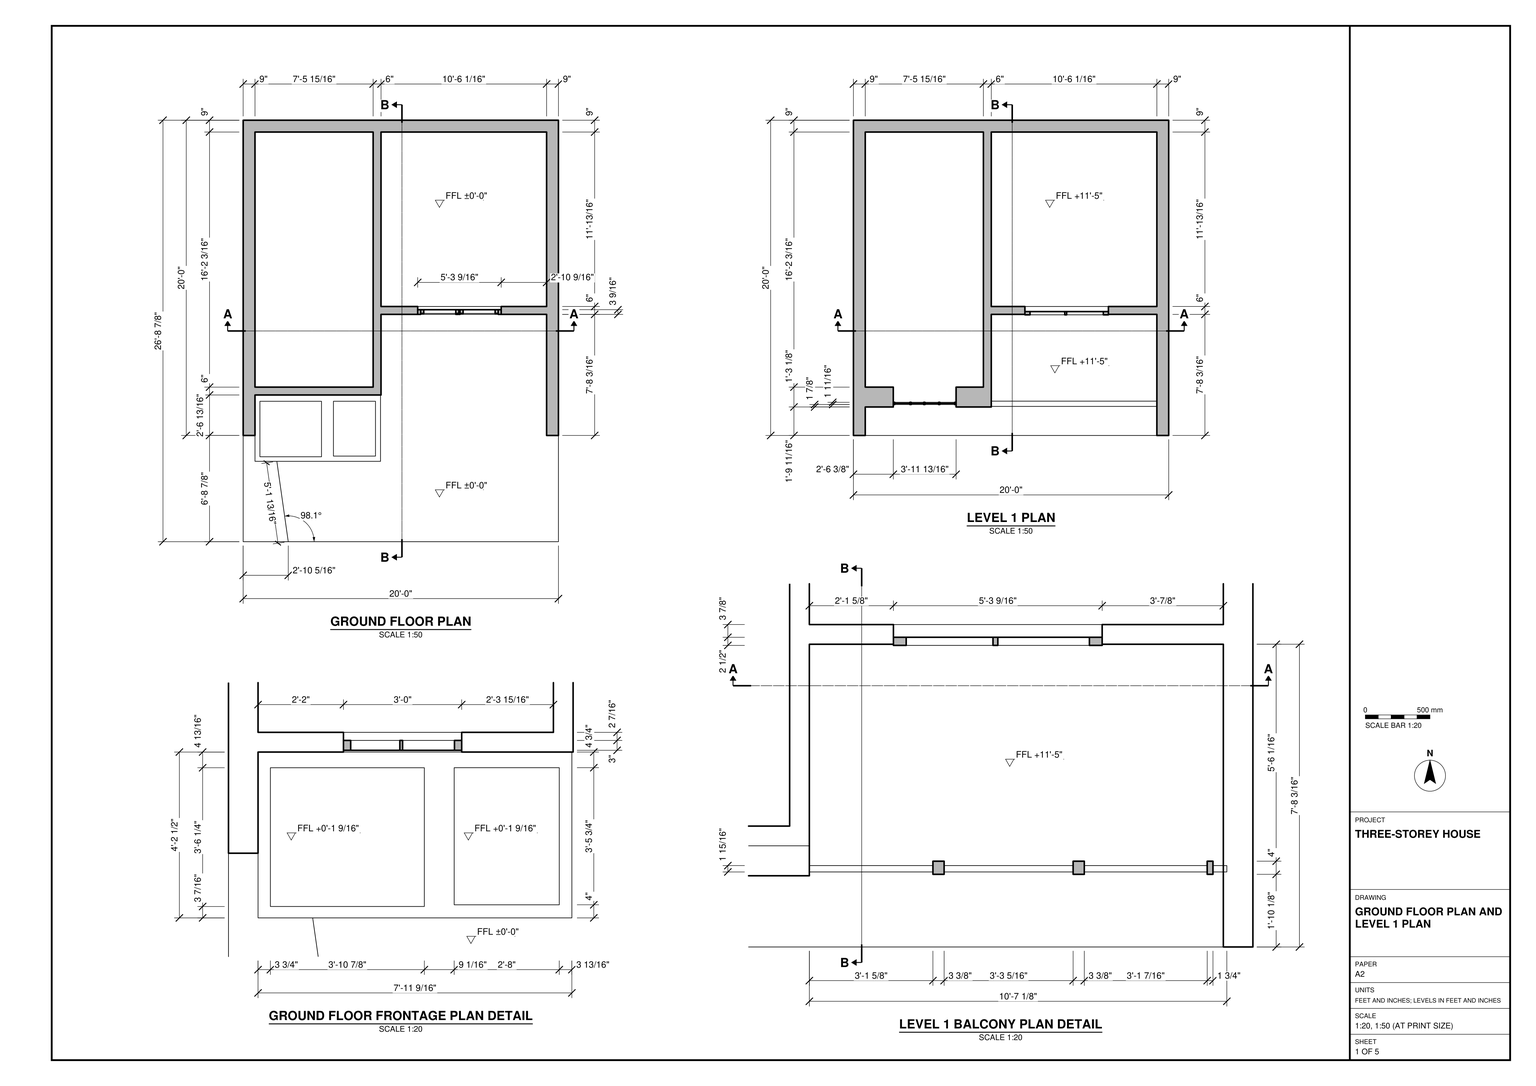
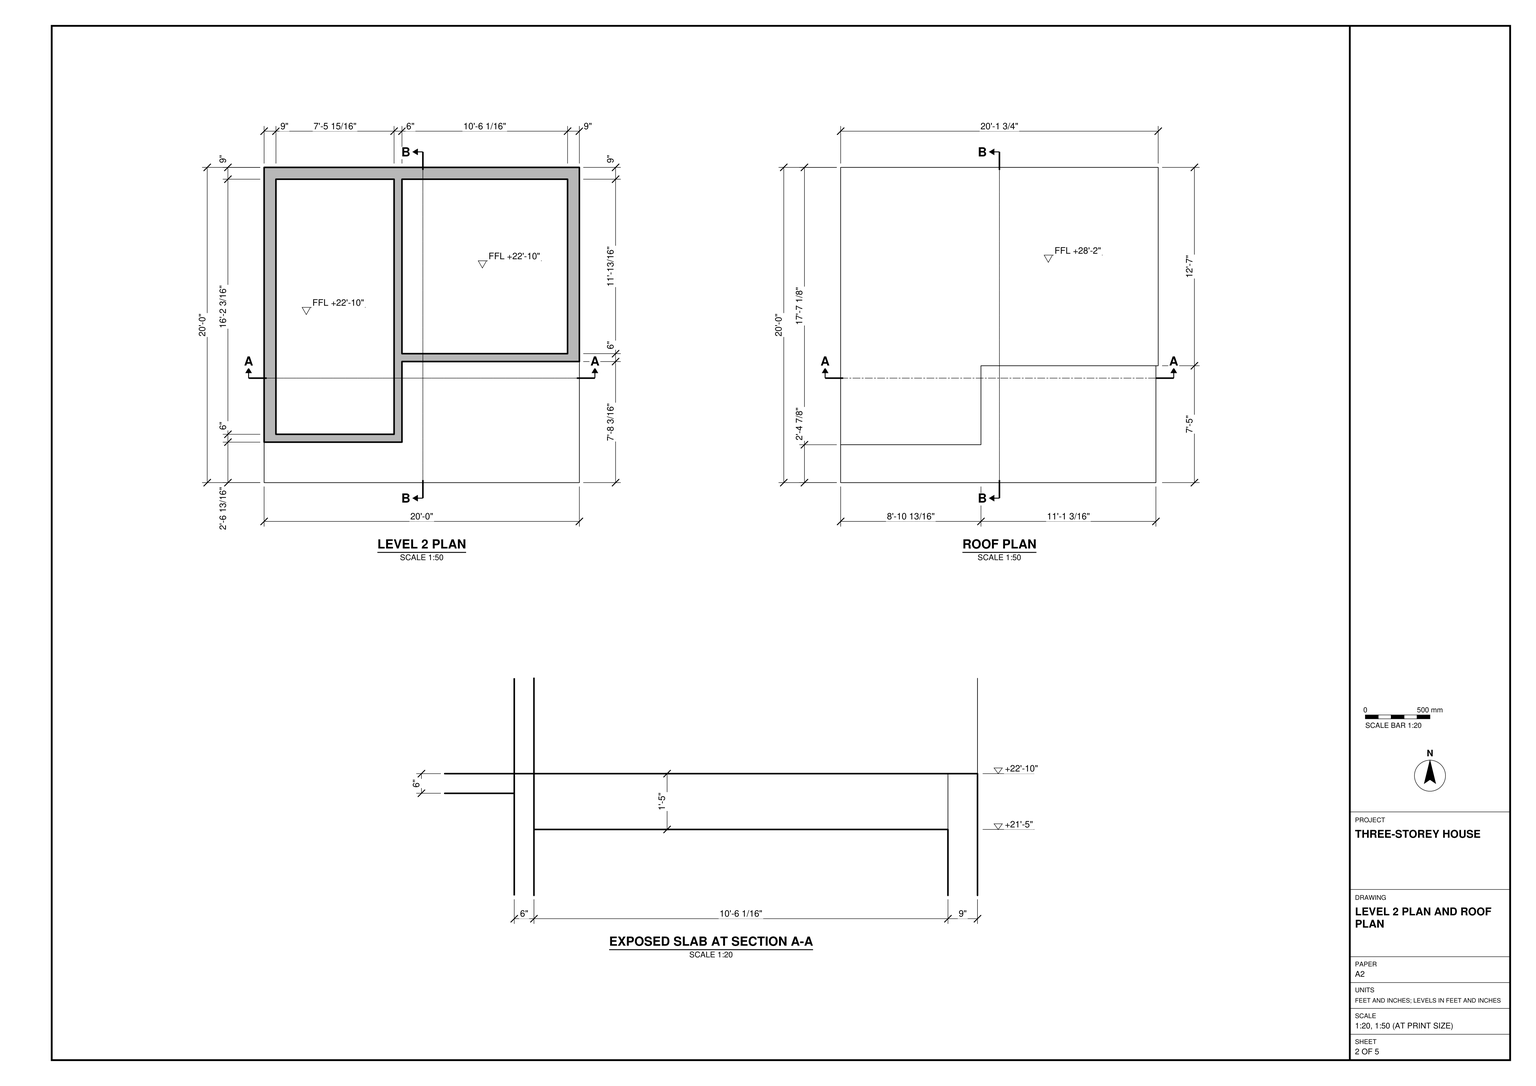
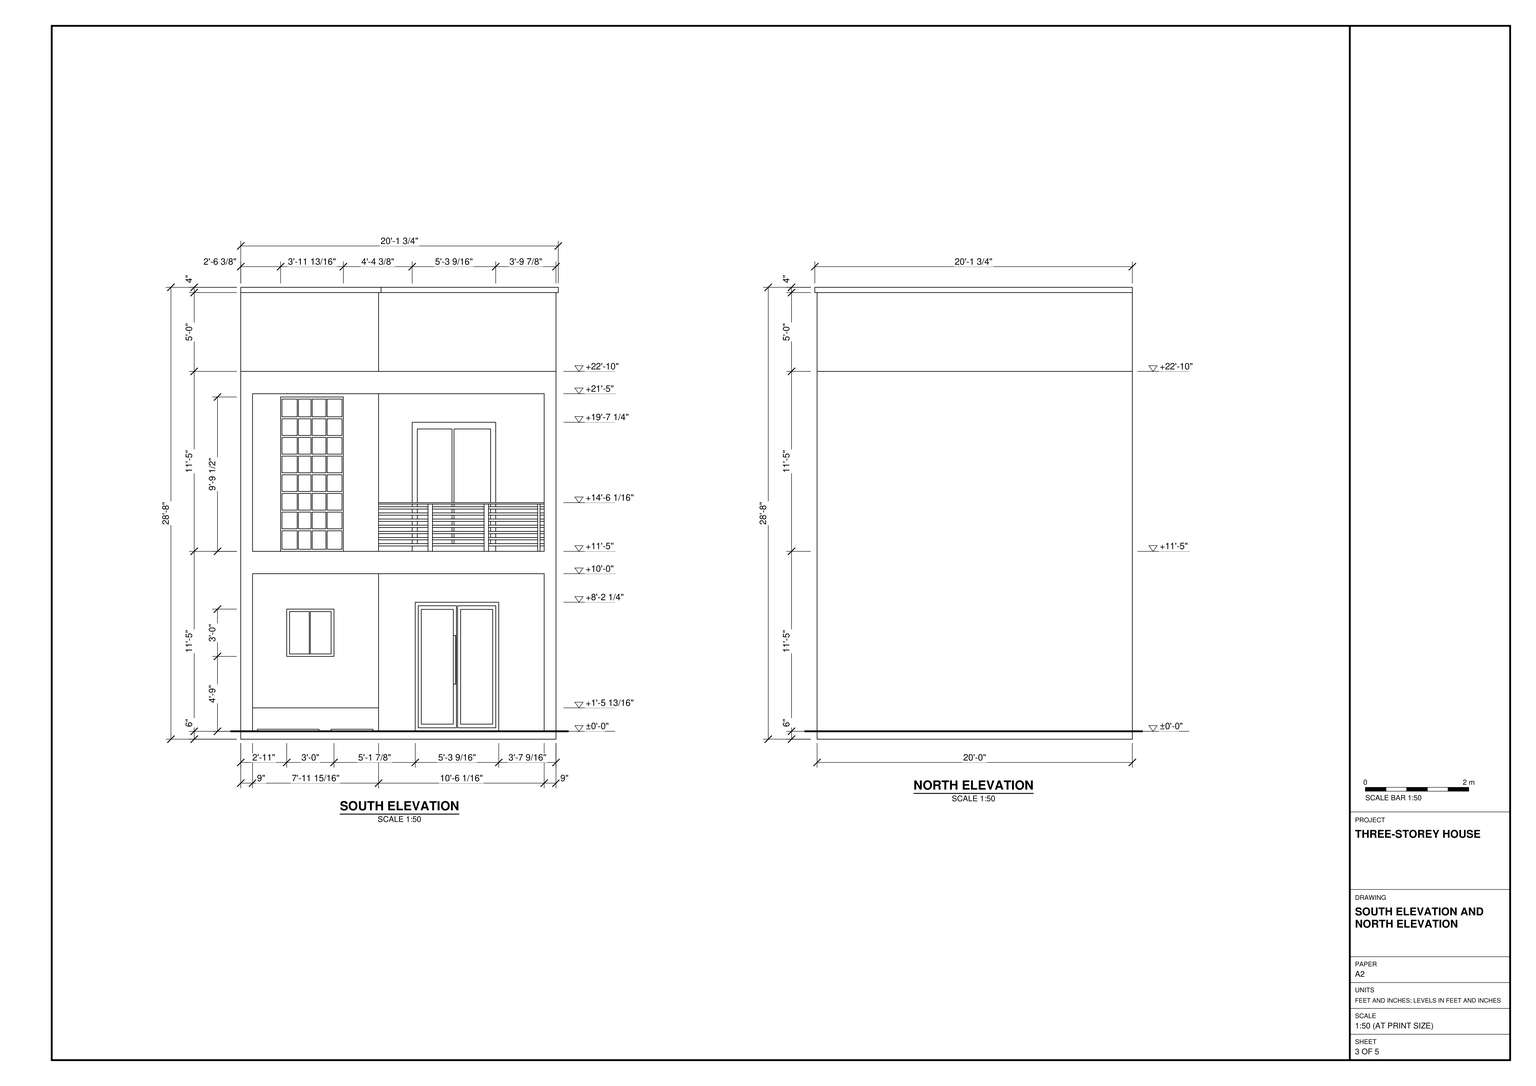
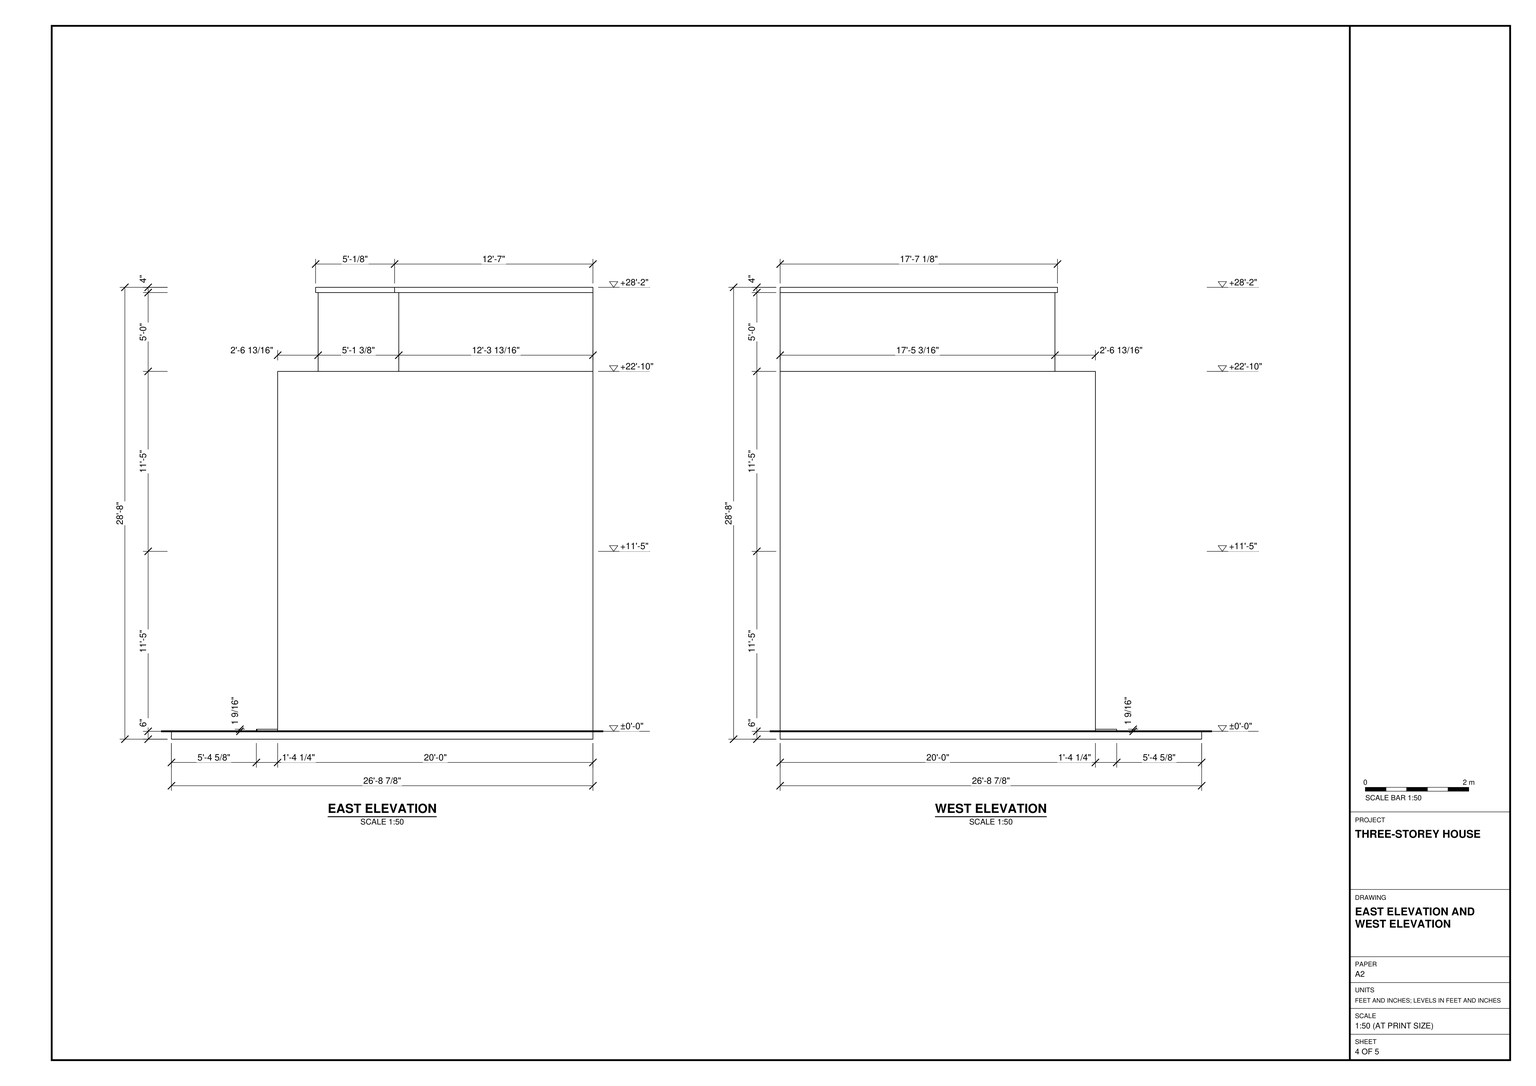
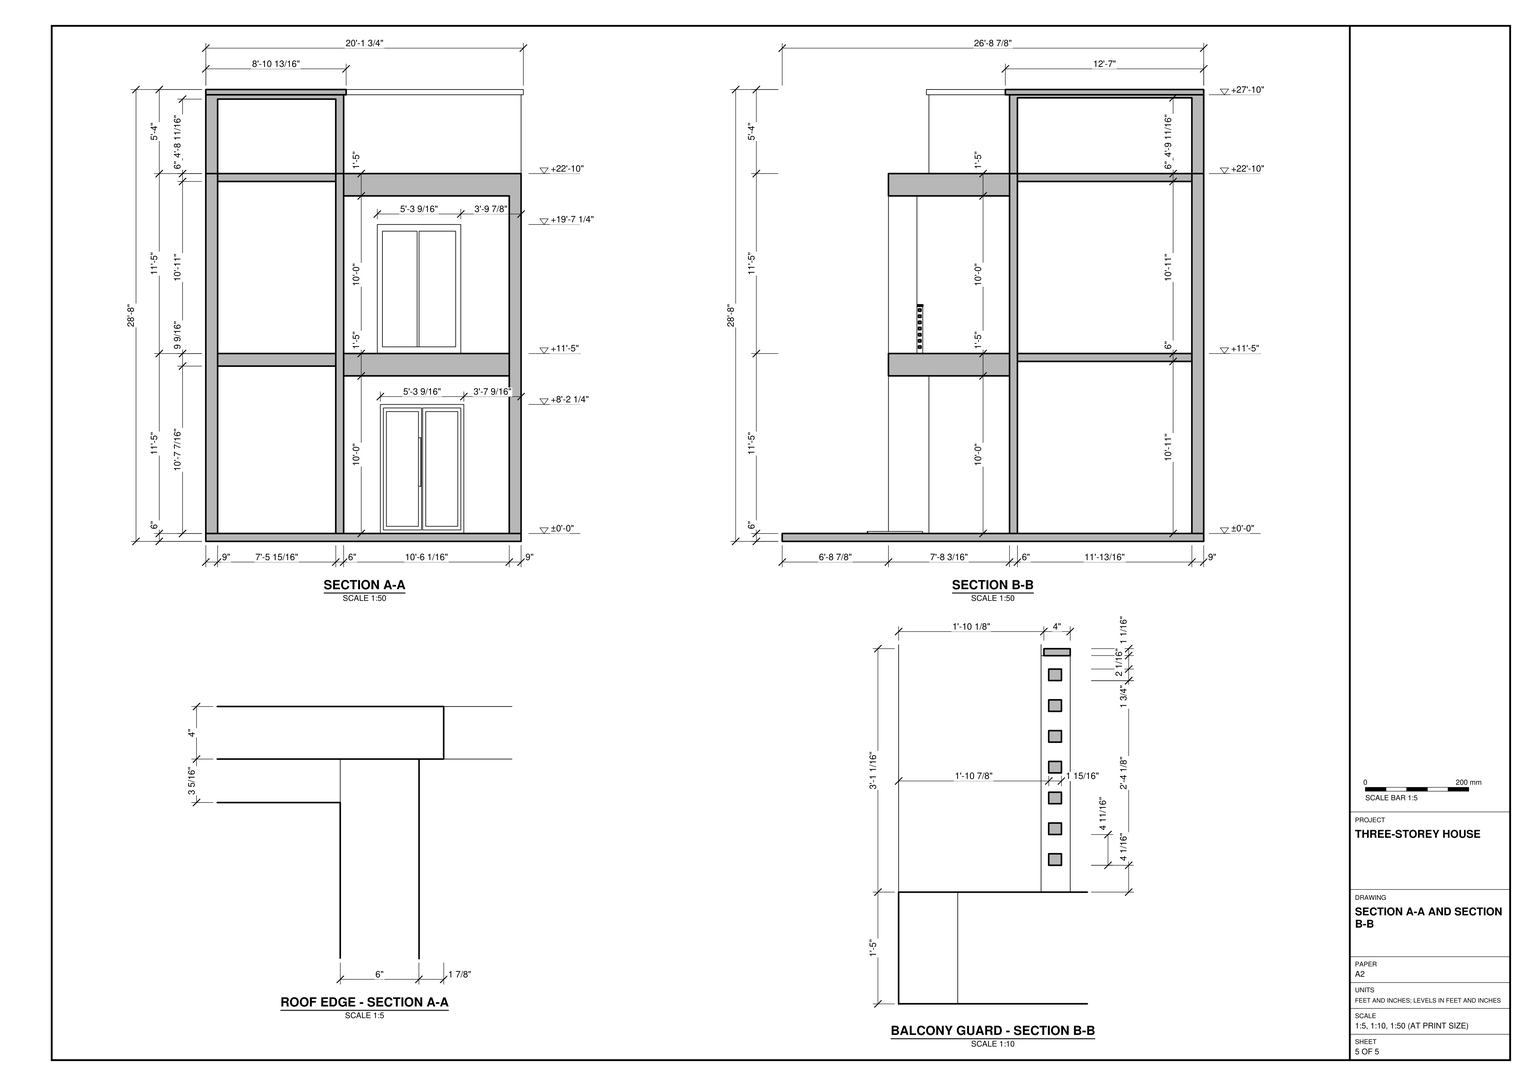
Build the three-storey house in SketchUp from task_files/diagram_01.pdf. Work in feet and inches. The overall model is 20'-1 3/4" wide, 26'-8 7/8" deep including the frontage, and 28'-8" high. Set the finished floor levels at ±0'-0", +11'-5" and +22'-10".

Lay out the narrow west bay and the wider east bay, with the west bay extending farther south. Follow the plans for the 9" side and rear walls and the 6" dividing walls. Carry the ground surface forward of the house and include the two rectangular areas within the border below the south window. Model the small divided window and paired entrance doors at ground level. Above them, place the tall gridded panel on the left and the recessed balcony with its glazed opening, posts and horizontal rails on the right. Use the section detail for the exposed slab and its deeper edge. Keep the north face continuous and fit the flat roof to the stepped outline of the low upper storey.

Keep walls, slabs, the roof, and any furniture or joinery pieces in separate groups or components; use components for repeated parts. Any decor or loose items shown may be suitable library components. Save one SketchUp model as output_files/three_storey_house_with_its_recessed_south_balcony.skp.

# SketchUp Ruby script. Lengths in inches.
U = 1.inch
M = Sketchup.active_model
def pt(a) = Geom::Point3d.new(a.map { |v| v * U })
def face(e, loops, mat)
  f = e.add_face(loops[0].map { |a| pt(a) })
  loops[1..].each { |l| e.add_face(l.map { |a| pt(a) }).erase! }
  f.material = f.back_material = mat if mat
  f
end
# faces: each face lists its corners as indices into pts; further lists are holes
def faces(e, pts, list, mat = nil) = list.each { |f| face(e, (f[0].is_a?(Array) ? f : [f]).map { |l| l.map { |i| pts[i] } }, mat) }
# xy, xz, yz: faces in a plane at the given z, y or x. An outline is a flat list of corners, or four numbers for a rectangle; further outlines are holes
def ring(l) = l.size == 4 ? [[l[0], l[1]], [l[2], l[1]], [l[2], l[3]], [l[0], l[3]]] : l.each_slice(2).to_a
def flat(e, list, mat, &to3) = list.each { |f| face(e, (f[0].is_a?(Array) ? f : [f]).map { |l| ring(l).map { |u, v| to3.(u, v) } }, mat) }
def xy(e, z, list, mat = nil) = flat(e, list, mat) { |x, y| [x, y, z] }
def xz(e, y, list, mat = nil) = flat(e, list, mat) { |x, z| [x, y, z] }
def yz(e, x, list, mat = nil) = flat(e, list, mat) { |y, z| [x, y, z] }
def lines(e, pts, list) = list.each { |a, b| e.add_line(pt(pts[a]), pt(pts[b])) }
# prism: a flat outline (further loops are holes) pulled along v
def prism(e, loops, v, mat = nil)
  f = face(e, loops, mat); d = Geom::Vector3d.new(v.map { |x| x * U })
  f.pushpull(f.normal.samedirection?(d) ? d.length : -d.length)
end
def box(e, o, s, mat = nil) = prism(e, [[o, [o[0] + s[0], o[1], o[2]], [o[0] + s[0], o[1] + s[1], o[2]], [o[0], o[1] + s[1], o[2]]]], [0, 0, s[2]], mat)
def at(x, y, z, deg = 0) = Geom::Transformation.translation(pt([x, y, z])) * Geom::Transformation.rotation(ORIGIN, Z_AXIS, deg.degrees)
def axes(o, x, y, z) = Geom::Transformation.new([*x, 0, *y, 0, *z, 0, *pt(o).to_a, 1])
def part(name) = M.definitions.add(name)
# library, detail: a bought-in or finely detailed component or shape, given as its bounding box
def library(name, o, s) = part(name).tap { |d| box(d.entities, o, s) }
def detail(e, o, s) = box(e.add_group.entities, o, s)
def put(e, d, t, mat = nil) = e.add_instance(d, t).tap { |i| i.material = mat if mat }
def group(e, t, mat = nil) = e.add_group.tap { |g| g.transformation = t; g.material = mat if mat }.entities
root = M.entities
M.materials.add("[Blacktop Old 02]").color = [143, 145, 145]
M.materials.add("[Cladding Stucco White]").color = [200, 200, 200]
M.materials.add("[Color M00]").color = [255, 255, 255]
M.materials.add("[Color M03]").color = [170, 170, 170]
M.materials.add("[Color M08]").color = [30, 30, 30]
M.materials.add("[Color M09]").color = [0, 0, 0]
M.materials.add("[Grass Dark Green]").color = [106, 157, 55]
M.materials.add("[Groundcover Rock Crushed 2 inch]").color = [130, 127, 128]
M.materials.add("[Stone Sandstone Ashlar Light]").color = [186, 182, 175]
M.materials.add("[Translucent Glass Gray]").color = [128, 128, 128]
M.materials["[Translucent Glass Gray]"].alpha = 0.5
M.materials.add("[Wood Bamboo]").color = [182, 120, 57]
c1 = part("Group\#2")
xy(c1.entities,0,[[0,0,103.125,4.1875]],"[Color M08]")
xy(c1.entities,6.3,[[49.1875,0,51.59,4.1875]])
xy(c1.entities,6.3,[[6.3,0,49.1875,4.1875],[51.59,0,96.82,4.1875]],"[Color M08]")
xy(c1.entities,115.32,[[6.3,0,49.1875,4.1875],[51.59,0,96.82,4.1875]],"[Color M08]")
xy(c1.entities,121.625,[[0,0,103.125,4.1875]],"[Color M08]")
xz(c1.entities,0,[[[0,0,103.125,121.625],[6.3,6.3,6.3,115.32,49.1875,115.32,49.1875,6.3,51.59,6.3,51.59,115.32,96.82,115.32,96.82,6.3]]],"[Color M08]")
xz(c1.entities,4.1875,[[[0,0,103.125,121.625],[6.3,6.3,96.82,6.3,96.82,115.32,51.59,115.32,51.59,6.3,49.1875,6.3,49.1875,115.32,6.3,115.32]]],"[Color M08]")
xz(c1.entities,4.1875,[[6.3,6.3,49.1875,115.32],[51.59,6.3,96.82,115.32]],"[Translucent Glass Gray]")
yz(c1.entities,0,[[0,0,4.1875,121.625]],"[Color M08]")
yz(c1.entities,6.3,[[0,6.3,4.1875,115.32]],"[Color M08]")
yz(c1.entities,49.1875,[[0,6.3,4.1875,115.32]],"[Color M08]")
yz(c1.entities,51.59,[[0,6.3,4.1875,115.32]],"[Color M08]")
yz(c1.entities,96.82,[[0,6.3,4.1875,115.32]],"[Color M08]")
yz(c1.entities,103.125,[[0,0,4.1875,121.625]],"[Color M08]")
xy(root,0,[[0,0,240,320.875]])
xy(root,6,[[12.76,64.65,59.63,106.9],[68.73,65.17,100.73,106.92],[[0,80.875,0,320.875,240,320.875,240,80.875,231,80.875,231,173.0625,196.42,173.0625,196.42,179.0625,231,179.0625,231,311.875,104.9375,311.875,104.9375,179.0625,132.86,179.0625,132.86,173.0625,104.9375,173.0625,104.9375,111.6875,9,111.6875,9,80.875],[9,117.6875,98.9375,311.875]],[9,117.6875,98.9375,311.875],[104.9375,179.0625,231,311.875]])
xy(root,6,[[34.32,0,240,0,240,80.875,231,80.875,231,173.0625,196.42,173.0625,196.42,179.0625,132.86,179.0625,132.86,173.0625,104.9375,173.0625,104.9375,111.6875,104.5625,111.6875,104.5625,61.1875,25.64,61.1875]],"[Cladding Stucco White]")
xy(root,6,[[0,0,34.32,0,25.64,61.1875,9,61.1875,9,80.875,0,80.875]],"[Grass Dark Green]")
xy(root,6,[[[9,61.1875,104.5625,111.6875],[12.76,64.65,59.63,106.9],[68.73,65.17,100.73,106.92]]],"[Groundcover Rock Crushed 2 inch]")
xy(root,7.5625,[[12.76,64.65,59.63,106.9],[68.73,65.17,100.73,106.92]])
xy(root,63.03,[[35.01,111.6875,71.01,117.6875]])
xy(root,99.03,[[35.01,111.6875,71.01,117.6875]])
xy(root,104.25,[[132.86,173.0625,196.42,179.0625]])
xy(root,126,[[9,80.875,9,111.6875,104.9375,111.6875,104.9375,173.0625,231,173.0625,231,80.875]],"[Color M03]")
xy(root,133.4375,[[9,117.6875,98.9375,311.875]])
xy(root,137,[[104.9375,179.0625,231,311.875]])
xy(root,143,[[9,102.5625,30.35,111.6875],[78.15,102.5625,104.9375,111.6875],[130.54,173.0625,194.1,179.0625],[104.9375,179.0625,231,311.875]])
xy(root,143,[[[9,80.875,231,80.875,231,173.0625,104.9375,173.0625,104.9375,102.5625,78.15,102.5625,78.15,117.6875,98.9375,117.6875,98.9375,311.875,9,311.875,9,117.6875,30.35,117.6875,30.35,102.5625,9,102.5625],[185.26,103,188.66,107],[142.57,103,145.97,107],[226.08,103,227.84,107]]],"[Blacktop Old 02]")
xy(root,143,[[142.57,103,145.97,107],[185.26,103,188.66,107],[226.08,103,227.84,107]],"[Color M08]")
xy(root,147.09,[[104.9375,103.73,231.5,105.66]],"[Color M09]")
xy(root,148.84,[[104.9375,103.73,231.5,105.66]],"[Color M09]")
xy(root,151.78,[[104.9375,103.73,231,105.66]],"[Color M09]")
xy(root,153.53,[[104.9375,103.73,231,105.66]],"[Color M09]")
xy(root,156.46,[[104.9375,103.73,231,105.66]],"[Color M09]")
xy(root,158.21,[[104.9375,103.73,231,105.66]],"[Color M09]")
xy(root,161.15,[[104.9375,103.73,231,105.66]],"[Color M09]")
xy(root,162.9,[[104.9375,103.73,231,105.66]],"[Color M09]")
xy(root,165.84,[[104.9375,103.73,231,105.66]],"[Color M09]")
xy(root,167.59,[[104.9375,103.73,231,105.66]],"[Color M09]")
xy(root,170.53,[[104.9375,103.73,232.0625,105.66]],"[Color M09]")
xy(root,172.28,[[104.9375,103.73,232.0625,105.66]],"[Color M09]")
xy(root,175.21,[[104.9375,103.73,231,105.66]],"[Color M09]")
xy(root,176.96,[[104.9375,103.73,231,105.66]],"[Color M09]")
xy(root,179,[[99.13,103,104.9375,107]],"[Color M00]")
xy(root,179,[[142.57,103,145.97,107],[185.26,103,188.66,107],[226.08,103,227.84,107]],"[Color M08]")
xy(root,179,[[104.9375,103,142.57,107],[145.97,103,185.26,107],[188.66,103,226.08,107],[227.84,103,231,107]],"[Color M09]")
xy(root,180.0625,[[99.13,103,231,107]],"[Color M08]")
xy(root,241.25,[[130.54,173.0625,194.1,179.0625]])
xy(root,260.5,[[30.35,102.5625,78.15,117.6875]])
xy(root,263,[[9,102.5625,104.9375,111.6875]])
xy(root,263,[[9,80.875,9,102.5625,104.9375,102.5625,104.9375,173.0625,231,173.0625,231,80.875]],"[Color M03]")
xy(root,274,[[9,117.6875,98.9375,311.875],[104.9375,179.0625,231,311.875]])
xy(root,280,[[[0,111.6875,0,320.875,240,320.875,240,173.0625,104.9375,173.0625,104.9375,111.6875],[9,117.6875,98.9375,311.875],[104.9375,179.0625,231,311.875]],[9,117.6875,98.9375,311.875],[104.9375,179.0625,231,311.875]])
xy(root,280,[[0,80.875,0,111.6875,104.9375,111.6875,104.9375,173.0625,240,173.0625,240,80.875]],"[Color M00]")
xy(root,336.6875,[[9,117.6875,98.9375,311.875]])
xy(root,337.6875,[[104.9375,179.0625,231,311.875]])
xy(root,340,[[0,109.75,0,111.6875,104.9375,111.6875,104.9375,173.0625,240,173.0625,240,320.875,241.75,320.875,241.75,169.875,106.8125,169.875,106.8125,109.75],[0,111.6875,0,320.875,240,320.875,240,173.0625,104.9375,173.0625,104.9375,111.6875]])
xy(root,344,[[0,109.75,106.8125,109.75,106.8125,169.875,241.75,169.875,241.75,320.875,0,320.875]])
xz(root,0,[[0,0,240,6]],"[Cladding Stucco White]")
xz(root,64.65,[[12.76,6,59.63,7.5625]])
xz(root,65.17,[[68.73,6,100.73,7.5625]])
xz(root,80.875,[[[0,6,9,6,9,126,231,126,231,6,240,6,240,280,0,280],[9,143,231,263]]])
xz(root,102.5625,[[9,143,30.35,143,30.35,260.5,78.15,260.5,78.15,143,104.9375,143,104.9375,263,9,263]],"[Color M03]")
xz(root,103,[[142.57,143,145.97,179],[185.26,143,188.66,179],[226.08,143,227.84,179]],"[Color M08]")
xz(root,103,[[99.13,179,231,180.0625]],"[Color M09]")
xz(root,103.73,[[104.9375,147.09,231.5,148.84],[104.9375,151.78,231,153.53],[104.9375,156.46,231,158.21],[104.9375,161.15,231,162.9],[104.9375,165.84,231,167.59],
  [104.9375,170.53,232.0625,172.28],[104.9375,175.21,231,176.96]],"[Color M09]")
xz(root,105.66,[[104.9375,147.09,231.5,148.84],[104.9375,151.78,231,153.53],[104.9375,156.46,231,158.21],[104.9375,161.15,231,162.9],[104.9375,165.84,231,167.59],
  [104.9375,170.53,232.0625,172.28],[104.9375,175.21,231,176.96]],"[Color M09]")
xz(root,106.9,[[12.76,6,59.63,7.5625]])
xz(root,106.92,[[68.73,6,100.73,7.5625]])
xz(root,107,[[142.57,143,145.97,179],[185.26,143,188.66,179],[226.08,143,227.84,179],[99.13,179,231,180.0625]],"[Color M08]")
xz(root,109.75,[[0,340,106.8125,344]])
xz(root,111.6875,[[9,263,104.9375,280]])
xz(root,111.6875,[[9,6,104.9375,23.83],[0,280,104.9375,340]],"[Color M03]")
xz(root,111.6875,[[[9,23.83,104.9375,126],[35.01,63.03,71.01,99.03]]],"[Stone Sandstone Ashlar Light]")
xz(root,117.6875,[[[9,6,98.9375,126],[35.01,63.03,71.01,99.03]],[9,126,98.9375,133.4375],[9,143,9,263,98.9375,263,98.9375,143,78.15,143,78.15,260.5,30.35,260.5,30.35,143],[9,263,98.9375,274],[9,274,98.9375,280],
  [9,280,98.9375,336.6875]])
xz(root,169.875,[[106.8125,340,241.75,344]])
xz(root,173.0625,[[104.9375,126,231,143],[104.9375,263,231,280]])
xz(root,173.0625,[[104.9375,6,132.86,6,132.86,104.25,196.42,104.25,196.42,6,231,6,231,126,104.9375,126],[104.9375,143,130.54,143,130.54,241.25,194.1,241.25,194.1,143,231,143,231,263,104.9375,263],[104.9375,280,240,340]],"[Color M03]")
xz(root,179.0625,[[104.9375,6,104.9375,126,231,126,231,6,196.42,6,196.42,104.25,132.86,104.25,132.86,6],[104.9375,126,231,137],[104.9375,137,231,143],[104.9375,143,104.9375,263,231,263,231,143,194.1,143,194.1,241.25,130.54,241.25,130.54,143],[104.9375,263,231,274],
  [104.9375,274,231,280],[104.9375,280,231,337.6875]])
xz(root,311.875,[[9,6,98.9375,133.4375],[104.9375,6,231,137],[9,133.4375,21.9375,143],[21.9375,133.4375,98.9375,143],[104.9375,137,167.97,143],
  [167.97,137,179.91,143],[179.91,137,231,143],[9,143,98.9375,274],[104.9375,143,231,274],[9,274,19.18,280],
  [19.18,274,34.8,280],[34.8,274,98.9375,280],[104.9375,274,116.87,280],[116.87,274,130.74,280],[130.74,274,231,280],
  [9,280,98.9375,336.6875],[104.9375,280,231,337.6875]])
xz(root,320.875,[[0,6,240,280],[0,340,241.75,344]])
xz(root,320.875,[[0,0,240,6]],"[Cladding Stucco White]")
xz(root,320.875,[[0,280,240,340]],"[Color M03]")
yz(root,0,[[80.875,6,320.875,280],[109.75,340,320.875,344]])
yz(root,0,[[0,0,320.875,6]],"[Cladding Stucco White]")
yz(root,0,[[111.6875,280,320.875,340]],"[Color M03]")
yz(root,9,[[117.6875,6,311.875,133.4375],[89.875,126,111.6875,143],[117.6875,133.4375,311.875,143],[117.6875,143,311.875,274],[117.6875,274,311.875,280],
  [117.6875,280,311.875,336.6875]])
yz(root,9,[[80.875,6,111.6875,126],[80.875,143,102.5625,263]],"[Color M03]")
yz(root,12.76,[[64.65,6,106.9,7.5625]])
yz(root,30.35,[[102.5625,143,117.6875,260.5]],"[Color M03]")
yz(root,35.01,[[111.6875,63.03,117.6875,99.03]])
yz(root,59.63,[[64.65,6,106.9,7.5625]])
yz(root,68.73,[[65.17,6,106.92,7.5625]])
yz(root,71.01,[[111.6875,63.03,117.6875,99.03]])
yz(root,78.15,[[102.5625,143,117.6875,260.5]],"[Color M03]")
yz(root,98.9375,[[117.6875,6,311.875,133.4375],[117.6875,133.4375,311.875,143],[117.6875,143,311.875,263],[117.6875,263,311.875,274],[117.6875,274,311.875,280],
  [117.6875,280,311.875,336.6875]])
yz(root,99.13,[[103,179,107,180.0625]],"[Color M00]")
yz(root,100.73,[[65.17,6,106.92,7.5625]])
yz(root,104.9375,[[179.0625,6,311.875,137],[111.6875,126,173.0625,143],[179.0625,137,311.875,143],[179.0625,143,311.875,274],[103.73,147.09,105.66,148.84],
  [103.73,151.78,105.66,153.53],[103.73,156.46,105.66,158.21],[103.73,161.15,105.66,162.9],[103.73,165.84,105.66,167.59],[103.73,170.53,105.66,172.28],
  [103.73,175.21,105.66,176.96],[111.6875,263,173.0625,280],[179.0625,274,311.875,280],[179.0625,280,311.875,337.6875]])
yz(root,104.9375,[[111.6875,6,173.0625,126],[107,143,173.0625,143,173.0625,263,102.5625,263,102.5625,179,107,179],[[102.5625,143,107,179],[103.73,147.09,105.66,148.84],[103.73,151.78,105.66,153.53],[103.73,156.46,105.66,158.21],[103.73,161.15,105.66,162.9],[103.73,165.84,105.66,167.59],[103.73,170.53,105.66,172.28],[103.73,175.21,105.66,176.96]],[111.6875,280,173.0625,340]],"[Color M03]")
yz(root,106.8125,[[109.75,340,169.875,344]])
yz(root,130.54,[[173.0625,143,179.0625,241.25]])
yz(root,132.86,[[173.0625,6,179.0625,104.25]])
yz(root,142.57,[[103,143,107,179]],"[Color M08]")
yz(root,145.97,[[103,143,107,179]],"[Color M08]")
yz(root,185.26,[[103,143,107,179]],"[Color M08]")
yz(root,188.66,[[103,143,107,179]],"[Color M08]")
yz(root,194.1,[[173.0625,143,179.0625,241.25]])
yz(root,196.42,[[173.0625,6,179.0625,104.25]])
yz(root,226.08,[[103,143,107,179]],"[Color M08]")
yz(root,227.84,[[103,143,107,179]],"[Color M08]")
yz(root,231,[[179.0625,6,311.875,137],[89.875,126,173.0625,143],[179.0625,137,311.875,143],[179.0625,143,311.875,274],[179.0625,274,311.875,280],
  [179.0625,280,311.875,337.6875]])
yz(root,231,[[80.875,6,173.0625,126],[[80.875,143,173.0625,263],[103,179,107,180.0625],[103.73,151.78,105.66,153.53],[103.73,156.46,105.66,158.21],[103.73,161.15,105.66,162.9],[103.73,165.84,105.66,167.59],[103.73,175.21,105.66,176.96]]],"[Color M03]")
yz(root,231.5,[[103.73,147.09,105.66,148.84]])
yz(root,232.0625,[[103.73,170.53,105.66,172.28]])
yz(root,240,[[80.875,6,320.875,280]])
yz(root,240,[[0,0,320.875,6]],"[Cladding Stucco White]")
yz(root,240,[[173.0625,280,320.875,340]],"[Color M03]")
yz(root,241.75,[[169.875,340,320.875,344]])
p = [[26.0625,311.875,340],[26.0625,311.875,336.6875],[9,117.6875,336.6875],[9,117.6875,340],[98.9375,117.6875,336.6875],[98.9375,117.6875,340],
  [98.9375,311.875,336.6875],[98.9375,311.875,340],[117.9375,311.875,340],[117.9375,311.875,337.6875],[104.9375,179.0625,337.6875],[104.9375,179.0625,340],
  [231,179.0625,337.6875],[231,179.0625,340]]
lines(root,p,[[0,1],[2,3],[4,5],[6,7],[8,9],[10,11],[12,13]])
g1 = group(root,at(132.86,173.0625,6))
xy(g1,0,[[0,0,63.5625,3.5625]],"[Wood Bamboo]")
xy(g1,2.6875,[[2.28,0.71,31.34,3.5625],[32.21,0.71,61.28,3.5625]])
xy(g1,2.6875,[[2.28,0,31.34,0.71],[32.21,0,61.28,0.71]],"[Wood Bamboo]")
xy(g1,5.44,[[4.62,0.71,29,3.5625],[34.55,0.71,58.95,3.5625]],"[Wood Bamboo]")
xy(g1,35.875,[[29,0,30.79,0.71]],"[Color M09]")
xy(g1,72.92,[[29,0,30.79,0.71]],"[Color M09]")
xy(g1,92.81,[[4.62,0.71,29,3.5625],[34.55,0.71,58.95,3.5625]],"[Wood Bamboo]")
xy(g1,95.5625,[[2.28,0.71,31.34,3.5625],[32.21,0.71,61.28,3.5625]])
xy(g1,95.5625,[[2.28,0,31.34,0.71],[32.21,0,61.28,0.71]],"[Wood Bamboo]")
xy(g1,98.25,[[0,0,63.5625,3.5625]],"[Wood Bamboo]")
xz(g1,0,[[29,35.875,30.79,72.92]],"[Color M09]")
xz(g1,0,[[[0,0,63.5625,98.25],[32.21,2.6875,61.28,95.5625],[2.28,2.6875,31.34,95.5625]]],"[Wood Bamboo]")
xz(g1,0.71,[[29,35.875,30.79,72.92]],"[Color M09]")
xz(g1,0.71,[[[2.28,2.6875,31.34,95.5625],[4.62,5.44,4.62,92.81,29,92.81,29,72.92,30.79,72.92,30.79,35.875,29,35.875,29,5.44]],[[32.21,2.6875,61.28,95.5625],[34.55,5.44,58.95,92.81]]],"[Wood Bamboo]")
xz(g1,3.5625,[[4.62,5.44,29,92.81],[34.55,5.44,58.95,92.81]],"[Translucent Glass Gray]")
xz(g1,3.5625,[[[0,0,63.5625,98.25],[32.21,2.6875,61.28,95.5625],[2.28,2.6875,31.34,95.5625]],[[2.28,2.6875,31.34,95.5625],[4.62,5.44,29,92.81]],[[32.21,2.6875,61.28,95.5625],[34.55,5.44,58.95,92.81]]],"[Wood Bamboo]")
yz(g1,0,[[0,0,3.5625,98.25]],"[Wood Bamboo]")
yz(g1,2.28,[[0.71,2.6875,3.5625,95.5625]])
yz(g1,2.28,[[0,2.6875,0.71,95.5625]],"[Wood Bamboo]")
yz(g1,4.62,[[0.71,5.44,3.5625,92.81]],"[Wood Bamboo]")
yz(g1,29,[[0,35.875,0.71,72.92]],"[Color M09]")
yz(g1,29,[[0.71,5.44,3.5625,92.81]],"[Wood Bamboo]")
yz(g1,30.79,[[0,35.875,0.71,72.92]],"[Color M09]")
yz(g1,31.34,[[0.71,2.6875,3.5625,95.5625]])
yz(g1,31.34,[[0,2.6875,0.71,95.5625]],"[Wood Bamboo]")
yz(g1,32.21,[[0.71,2.6875,3.5625,95.5625]])
yz(g1,32.21,[[0,2.6875,0.71,95.5625]],"[Wood Bamboo]")
yz(g1,34.55,[[0.71,5.44,3.5625,92.81]],"[Wood Bamboo]")
yz(g1,58.95,[[0.71,5.44,3.5625,92.81]],"[Wood Bamboo]")
yz(g1,61.28,[[0.71,2.6875,3.5625,95.5625]])
yz(g1,61.28,[[0,2.6875,0.71,95.5625]],"[Wood Bamboo]")
yz(g1,63.5625,[[0,0,3.5625,98.25]],"[Wood Bamboo]")
put(root,c1,axes([130.54,172.72,143],[0.61636,0,0],[0,0.59,0],[0,0,0.80781]))
put(root,c1,axes([35.01,115.23,63.03],[0.34909,0,0],[0,-0.7196,0],[0,0,0.29599]))
g2 = group(root,at(30.35,104.4375,143))
xy(g2,0,[[0,0,47.8,0.83],[0,0.83,47.8,1.69]],"[Color M08]")
xy(g2,1.57,[[1.03,0,12.66,0.83],[13.58,0,23.16,0.83],[24.08,0,34.5,0.83],[35.42,0,46.77,0.83],[1.03,0.83,12.66,1.69],
  [13.58,0.83,23.16,1.69],[24.08,0.83,34.5,1.69],[35.42,0.83,46.77,1.69]],"[Color M08]")
xy(g2,15.65,[[1.03,0,12.66,0.83],[13.58,0,23.16,0.83],[24.08,0,34.5,0.83],[35.42,0,46.77,0.83],[1.03,0.83,12.66,1.69],
  [13.58,0.83,23.16,1.69],[24.08,0.83,34.5,1.69],[35.42,0.83,46.77,1.69]],"[Color M08]")
xy(g2,17.15,[[1.03,0,12.66,0.83],[13.58,0,23.16,0.83],[24.08,0,34.5,0.83],[35.42,0,46.77,0.83],[1.03,0.83,12.66,1.69],
  [13.58,0.83,23.16,1.69],[24.08,0.83,34.5,1.69],[35.42,0.83,46.77,1.69]],"[Color M08]")
xy(g2,29.86,[[1.03,0,12.66,0.83],[13.58,0,23.16,0.83],[24.08,0,34.5,0.83],[35.42,0,46.77,0.83],[1.03,0.83,12.66,1.69],
  [13.58,0.83,23.16,1.69],[24.08,0.83,34.5,1.69],[35.42,0.83,46.77,1.69]],"[Color M08]")
xy(g2,31.37,[[1.03,0,12.66,0.83],[13.58,0,23.16,0.83],[24.08,0,34.5,0.83],[35.42,0,46.77,0.83],[1.03,0.83,12.66,1.69],
  [13.58,0.83,23.16,1.69],[24.08,0.83,34.5,1.69],[35.42,0.83,46.77,1.69]],"[Color M08]")
xy(g2,44.07,[[1.03,0,12.66,0.83],[13.58,0,23.16,0.83],[24.08,0,34.5,0.83],[35.42,0,46.77,0.83],[1.03,0.83,12.66,1.69],
  [13.58,0.83,23.16,1.69],[24.08,0.83,34.5,1.69],[35.42,0.83,46.77,1.69]],"[Color M08]")
xy(g2,45.58,[[1.03,0,12.66,0.83],[13.58,0,23.16,0.83],[24.08,0,34.5,0.83],[35.42,0,46.77,0.83],[1.03,0.83,12.66,1.69],
  [13.58,0.83,23.16,1.69],[24.08,0.83,34.5,1.69],[35.42,0.83,46.77,1.69]],"[Color M08]")
xy(g2,58.28,[[1.03,0,12.66,0.83],[13.58,0,23.16,0.83],[24.08,0,34.5,0.83],[35.42,0,46.77,0.83],[1.03,0.83,12.66,1.69],
  [13.58,0.83,23.16,1.69],[24.08,0.83,34.5,1.69],[35.42,0.83,46.77,1.69]],"[Color M08]")
xy(g2,59.79,[[1.03,0,12.66,0.83],[13.58,0,23.16,0.83],[24.08,0,34.5,0.83],[35.42,0,46.77,0.83],[1.03,0.83,12.66,1.69],
  [13.58,0.83,23.16,1.69],[24.08,0.83,34.5,1.69],[35.42,0.83,46.77,1.69]],"[Color M08]")
xy(g2,72.5,[[1.03,0,12.66,0.83],[13.58,0,23.16,0.83],[24.08,0,34.5,0.83],[35.42,0,46.77,0.83],[1.03,0.83,12.66,1.69],
  [13.58,0.83,23.16,1.69],[24.08,0.83,34.5,1.69],[35.42,0.83,46.77,1.69]],"[Color M08]")
xy(g2,74,[[1.03,0,12.66,0.83],[13.58,0,23.16,0.83],[24.08,0,34.5,0.83],[35.42,0,46.77,0.83],[1.03,0.83,12.66,1.69],
  [13.58,0.83,23.16,1.69],[24.08,0.83,34.5,1.69],[35.42,0.83,46.77,1.69]],"[Color M08]")
xy(g2,86.71,[[1.03,0,12.66,0.83],[13.58,0,23.16,0.83],[24.08,0,34.5,0.83],[35.42,0,46.77,0.83],[1.03,0.83,12.66,1.69],
  [13.58,0.83,23.16,1.69],[24.08,0.83,34.5,1.69],[35.42,0.83,46.77,1.69]],"[Color M08]")
xy(g2,88.22,[[1.03,0,12.66,0.83],[13.58,0,23.16,0.83],[24.08,0,34.5,0.83],[35.42,0,46.77,0.83],[1.03,0.83,12.66,1.69],
  [13.58,0.83,23.16,1.69],[24.08,0.83,34.5,1.69],[35.42,0.83,46.77,1.69]],"[Color M08]")
xy(g2,100.92,[[1.03,0,12.66,0.83],[13.58,0,23.16,0.83],[24.08,0,34.5,0.83],[35.42,0,46.77,0.83],[1.03,0.83,12.66,1.69],
  [13.58,0.83,23.16,1.69],[24.08,0.83,34.5,1.69],[35.42,0.83,46.77,1.69]],"[Color M08]")
xy(g2,102.43,[[1.03,0,12.66,0.83],[13.58,0,23.16,0.83],[24.08,0,34.5,0.83],[35.42,0,46.77,0.83],[1.03,0.83,12.66,1.69],
  [13.58,0.83,23.16,1.69],[24.08,0.83,34.5,1.69],[35.42,0.83,46.77,1.69]],"[Color M08]")
xy(g2,115.93,[[1.03,0,12.66,0.83],[13.58,0,23.16,0.83],[24.08,0,34.5,0.83],[35.42,0,46.77,0.83],[1.03,0.83,12.66,1.69],
  [13.58,0.83,23.16,1.69],[24.08,0.83,34.5,1.69],[35.42,0.83,46.77,1.69]],"[Color M08]")
xy(g2,117.5,[[0,0,47.8,0.83],[0,0.83,47.8,1.69]],"[Color M08]")
xz(g2,0,[[[0,0,47.8,117.5],[1.03,1.57,12.66,15.65],[35.42,1.57,46.77,15.65],[1.03,102.43,12.66,115.93],[35.42,102.43,46.77,115.93],[1.03,88.22,12.66,100.92],[1.03,17.15,12.66,29.86],[1.03,31.37,12.66,44.07],[1.03,45.58,12.66,58.28],[1.03,59.79,12.66,72.5],[1.03,74,12.66,86.71],[24.08,1.57,34.5,15.65],[35.42,88.22,46.77,100.92],[35.42,74,46.77,86.71],[35.42,45.58,46.77,58.28],[35.42,59.79,46.77,72.5],[35.42,31.37,46.77,44.07],[35.42,17.15,46.77,29.86],[24.08,102.43,34.5,115.93],[13.58,1.57,23.16,15.65],[24.08,88.22,34.5,100.92],[24.08,74,34.5,86.71],[24.08,17.15,34.5,29.86],[24.08,31.37,34.5,44.07],[24.08,59.79,34.5,72.5],[24.08,45.58,34.5,58.28],[13.58,102.43,23.16,115.93],[13.58,88.22,23.16,100.92],[13.58,74,23.16,86.71],[13.58,17.15,23.16,29.86],[13.58,59.79,23.16,72.5],[13.58,31.37,23.16,44.07],[13.58,45.58,23.16,58.28]]],"[Color M08]")
xz(g2,0.83,[[[0,0,47.8,117.5],[1.03,1.57,12.66,15.65],[35.42,1.57,46.77,15.65],[1.03,102.43,12.66,115.93],[35.42,102.43,46.77,115.93],[1.03,88.22,12.66,100.92],[1.03,17.15,12.66,29.86],[1.03,31.37,12.66,44.07],[1.03,45.58,12.66,58.28],[1.03,59.79,12.66,72.5],[1.03,74,12.66,86.71],[24.08,1.57,34.5,15.65],[35.42,88.22,46.77,100.92],[35.42,74,46.77,86.71],[35.42,45.58,46.77,58.28],[35.42,59.79,46.77,72.5],[35.42,31.37,46.77,44.07],[35.42,17.15,46.77,29.86],[24.08,102.43,34.5,115.93],[13.58,1.57,23.16,15.65],[24.08,88.22,34.5,100.92],[24.08,74,34.5,86.71],[24.08,17.15,34.5,29.86],[24.08,31.37,34.5,44.07],[24.08,59.79,34.5,72.5],[24.08,45.58,34.5,58.28],[13.58,102.43,23.16,115.93],[13.58,88.22,23.16,100.92],[13.58,74,23.16,86.71],[13.58,17.15,23.16,29.86],[13.58,59.79,23.16,72.5],[13.58,31.37,23.16,44.07],[13.58,45.58,23.16,58.28]]],"[Color M08]")
xz(g2,0.83,[[1.03,1.57,12.66,15.65],[13.58,1.57,23.16,15.65],[24.08,1.57,34.5,15.65],[35.42,1.57,46.77,15.65],[1.03,17.15,12.66,29.86],
  [13.58,17.15,23.16,29.86],[24.08,17.15,34.5,29.86],[35.42,17.15,46.77,29.86],[1.03,31.37,12.66,44.07],[13.58,31.37,23.16,44.07],
  [24.08,31.37,34.5,44.07],[35.42,31.37,46.77,44.07],[1.03,45.58,12.66,58.28],[13.58,45.58,23.16,58.28],[24.08,45.58,34.5,58.28],
  [35.42,45.58,46.77,58.28],[1.03,59.79,12.66,72.5],[13.58,59.79,23.16,72.5],[24.08,59.79,34.5,72.5],[35.42,59.79,46.77,72.5],
  [1.03,74,12.66,86.71],[13.58,74,23.16,86.71],[24.08,74,34.5,86.71],[35.42,74,46.77,86.71],[1.03,88.22,12.66,100.92],
  [13.58,88.22,23.16,100.92],[24.08,88.22,34.5,100.92],[35.42,88.22,46.77,100.92],[1.03,102.43,12.66,115.93],[13.58,102.43,23.16,115.93],
  [24.08,102.43,34.5,115.93],[35.42,102.43,46.77,115.93]],"[Translucent Glass Gray]")
xz(g2,1.69,[[[0,0,47.8,117.5],[1.03,1.57,12.66,15.65],[35.42,1.57,46.77,15.65],[1.03,102.43,12.66,115.93],[35.42,102.43,46.77,115.93],[1.03,88.22,12.66,100.92],[1.03,17.15,12.66,29.86],[1.03,31.37,12.66,44.07],[1.03,45.58,12.66,58.28],[1.03,59.79,12.66,72.5],[1.03,74,12.66,86.71],[24.08,1.57,34.5,15.65],[35.42,88.22,46.77,100.92],[35.42,74,46.77,86.71],[35.42,45.58,46.77,58.28],[35.42,59.79,46.77,72.5],[35.42,31.37,46.77,44.07],[35.42,17.15,46.77,29.86],[24.08,102.43,34.5,115.93],[13.58,1.57,23.16,15.65],[24.08,88.22,34.5,100.92],[24.08,74,34.5,86.71],[24.08,17.15,34.5,29.86],[24.08,31.37,34.5,44.07],[24.08,59.79,34.5,72.5],[24.08,45.58,34.5,58.28],[13.58,102.43,23.16,115.93],[13.58,88.22,23.16,100.92],[13.58,74,23.16,86.71],[13.58,17.15,23.16,29.86],[13.58,59.79,23.16,72.5],[13.58,31.37,23.16,44.07],[13.58,45.58,23.16,58.28]]],"[Color M08]")
yz(g2,0,[[0,0,0.83,117.5],[0.83,0,1.69,117.5]],"[Color M08]")
yz(g2,1.03,[[0,1.57,0.83,15.65],[0.83,1.57,1.69,15.65],[0,17.15,0.83,29.86],[0.83,17.15,1.69,29.86],[0,31.37,0.83,44.07],
  [0.83,31.37,1.69,44.07],[0,45.58,0.83,58.28],[0.83,45.58,1.69,58.28],[0,59.79,0.83,72.5],[0.83,59.79,1.69,72.5],
  [0,74,0.83,86.71],[0.83,74,1.69,86.71],[0,88.22,0.83,100.92],[0.83,88.22,1.69,100.92],[0,102.43,0.83,115.93],
  [0.83,102.43,1.69,115.93]],"[Color M08]")
yz(g2,12.66,[[0,1.57,0.83,15.65],[0.83,1.57,1.69,15.65],[0,17.15,0.83,29.86],[0.83,17.15,1.69,29.86],[0,31.37,0.83,44.07],
  [0.83,31.37,1.69,44.07],[0,45.58,0.83,58.28],[0.83,45.58,1.69,58.28],[0,59.79,0.83,72.5],[0.83,59.79,1.69,72.5],
  [0,74,0.83,86.71],[0.83,74,1.69,86.71],[0,88.22,0.83,100.92],[0.83,88.22,1.69,100.92],[0,102.43,0.83,115.93],
  [0.83,102.43,1.69,115.93]],"[Color M08]")
yz(g2,13.58,[[0,1.57,0.83,15.65],[0.83,1.57,1.69,15.65],[0,17.15,0.83,29.86],[0.83,17.15,1.69,29.86],[0,31.37,0.83,44.07],
  [0.83,31.37,1.69,44.07],[0,45.58,0.83,58.28],[0.83,45.58,1.69,58.28],[0,59.79,0.83,72.5],[0.83,59.79,1.69,72.5],
  [0,74,0.83,86.71],[0.83,74,1.69,86.71],[0,88.22,0.83,100.92],[0.83,88.22,1.69,100.92],[0,102.43,0.83,115.93],
  [0.83,102.43,1.69,115.93]],"[Color M08]")
yz(g2,23.16,[[0,1.57,0.83,15.65],[0.83,1.57,1.69,15.65],[0,17.15,0.83,29.86],[0.83,17.15,1.69,29.86],[0,31.37,0.83,44.07],
  [0.83,31.37,1.69,44.07],[0,45.58,0.83,58.28],[0.83,45.58,1.69,58.28],[0,59.79,0.83,72.5],[0.83,59.79,1.69,72.5],
  [0,74,0.83,86.71],[0.83,74,1.69,86.71],[0,88.22,0.83,100.92],[0.83,88.22,1.69,100.92],[0,102.43,0.83,115.93],
  [0.83,102.43,1.69,115.93]],"[Color M08]")
yz(g2,24.08,[[0,1.57,0.83,15.65],[0.83,1.57,1.69,15.65],[0,17.15,0.83,29.86],[0.83,17.15,1.69,29.86],[0,31.37,0.83,44.07],
  [0.83,31.37,1.69,44.07],[0,45.58,0.83,58.28],[0.83,45.58,1.69,58.28],[0,59.79,0.83,72.5],[0.83,59.79,1.69,72.5],
  [0,74,0.83,86.71],[0.83,74,1.69,86.71],[0,88.22,0.83,100.92],[0.83,88.22,1.69,100.92],[0,102.43,0.83,115.93],
  [0.83,102.43,1.69,115.93]],"[Color M08]")
yz(g2,34.5,[[0,1.57,0.83,15.65],[0.83,1.57,1.69,15.65],[0,17.15,0.83,29.86],[0.83,17.15,1.69,29.86],[0,31.37,0.83,44.07],
  [0.83,31.37,1.69,44.07],[0,45.58,0.83,58.28],[0.83,45.58,1.69,58.28],[0,59.79,0.83,72.5],[0.83,59.79,1.69,72.5],
  [0,74,0.83,86.71],[0.83,74,1.69,86.71],[0,88.22,0.83,100.92],[0.83,88.22,1.69,100.92],[0,102.43,0.83,115.93],
  [0.83,102.43,1.69,115.93]],"[Color M08]")
yz(g2,35.42,[[0,1.57,0.83,15.65],[0.83,1.57,1.69,15.65],[0,17.15,0.83,29.86],[0.83,17.15,1.69,29.86],[0,31.37,0.83,44.07],
  [0.83,31.37,1.69,44.07],[0,45.58,0.83,58.28],[0.83,45.58,1.69,58.28],[0,59.79,0.83,72.5],[0.83,59.79,1.69,72.5],
  [0,74,0.83,86.71],[0.83,74,1.69,86.71],[0,88.22,0.83,100.92],[0.83,88.22,1.69,100.92],[0,102.43,0.83,115.93],
  [0.83,102.43,1.69,115.93]],"[Color M08]")
yz(g2,46.77,[[0,1.57,0.83,15.65],[0.83,1.57,1.69,15.65],[0,17.15,0.83,29.86],[0.83,17.15,1.69,29.86],[0,31.37,0.83,44.07],
  [0.83,31.37,1.69,44.07],[0,45.58,0.83,58.28],[0.83,45.58,1.69,58.28],[0,59.79,0.83,72.5],[0.83,59.79,1.69,72.5],
  [0,74,0.83,86.71],[0.83,74,1.69,86.71],[0,88.22,0.83,100.92],[0.83,88.22,1.69,100.92],[0,102.43,0.83,115.93],
  [0.83,102.43,1.69,115.93]],"[Color M08]")
yz(g2,47.8,[[0,0,0.83,117.5],[0.83,0,1.69,117.5]],"[Color M08]")
